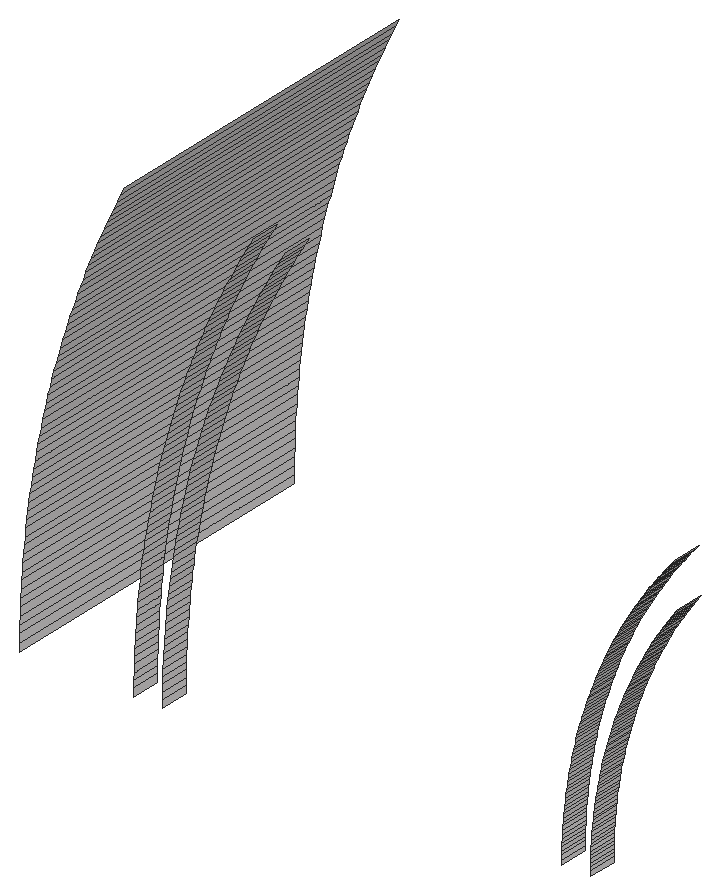
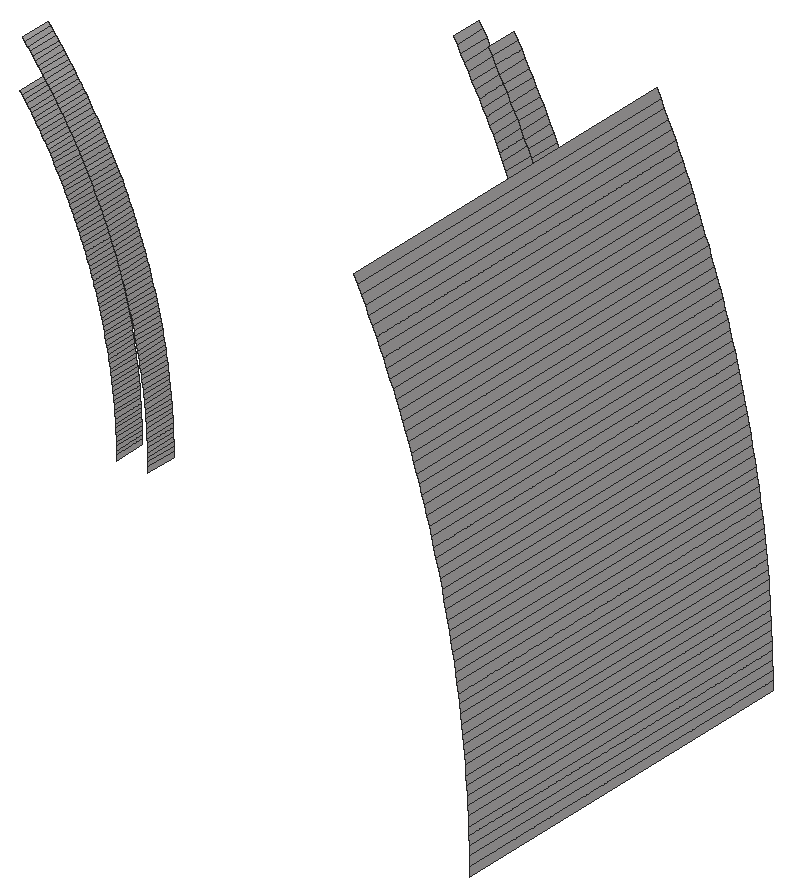
# SketchUp Ruby script. Lengths in inches.
U = 1.inch
M = Sketchup.active_model
def pt(a) = Geom::Point3d.new(a.map { |v| v * U })
def face(e, loops, mat)
  f = e.add_face(loops[0].map { |a| pt(a) })
  loops[1..].each { |l| e.add_face(l.map { |a| pt(a) }).erase! }
  f.material = f.back_material = mat if mat
  f
end
# faces: each face lists its corners as indices into pts; further lists are holes
def faces(e, pts, list, mat = nil) = list.each { |f| face(e, (f[0].is_a?(Array) ? f : [f]).map { |l| l.map { |i| pts[i] } }, mat) }
# xy, xz, yz: faces in a plane at the given z, y or x. An outline is a flat list of corners, or four numbers for a rectangle; further outlines are holes
def ring(l) = l.size == 4 ? [[l[0], l[1]], [l[2], l[1]], [l[2], l[3]], [l[0], l[3]]] : l.each_slice(2).to_a
def flat(e, list, mat, &to3) = list.each { |f| face(e, (f[0].is_a?(Array) ? f : [f]).map { |l| ring(l).map { |u, v| to3.(u, v) } }, mat) }
def xy(e, z, list, mat = nil) = flat(e, list, mat) { |x, y| [x, y, z] }
def xz(e, y, list, mat = nil) = flat(e, list, mat) { |x, z| [x, y, z] }
def yz(e, x, list, mat = nil) = flat(e, list, mat) { |y, z| [x, y, z] }
def lines(e, pts, list) = list.each { |a, b| e.add_line(pt(pts[a]), pt(pts[b])) }
# prism: a flat outline (further loops are holes) pulled along v
def prism(e, loops, v, mat = nil)
  f = face(e, loops, mat); d = Geom::Vector3d.new(v.map { |x| x * U })
  f.pushpull(f.normal.samedirection?(d) ? d.length : -d.length)
end
def box(e, o, s, mat = nil) = prism(e, [[o, [o[0] + s[0], o[1], o[2]], [o[0] + s[0], o[1] + s[1], o[2]], [o[0], o[1] + s[1], o[2]]]], [0, 0, s[2]], mat)
def at(x, y, z, deg = 0) = Geom::Transformation.translation(pt([x, y, z])) * Geom::Transformation.rotation(ORIGIN, Z_AXIS, deg.degrees)
def axes(o, x, y, z) = Geom::Transformation.new([*x, 0, *y, 0, *z, 0, *pt(o).to_a, 1])
def part(name) = M.definitions.add(name)
# library, detail: a bought-in or finely detailed component or shape, given as its bounding box
def library(name, o, s) = part(name).tap { |d| box(d.entities, o, s) }
def detail(e, o, s) = box(e.add_group.entities, o, s)
def put(e, d, t, mat = nil) = e.add_instance(d, t).tap { |i| i.material = mat if mat }
def group(e, t, mat = nil) = e.add_group.tap { |g| g.transformation = t; g.material = mat if mat }.entities
root = M.entities
M.materials.add("[Quartz Light Brown]").color = [215, 212, 212]
yz(root,0,[[38,84,50,84.28],[38,84.28,50,84.57]],"[Quartz Light Brown]")
yz(root,4,[[38,83.99,39,84.25],[38,84.25,39,84.5]],"[Quartz Light Brown]")
yz(root,4.02,[[38,85.01,39,85.26]],"[Quartz Light Brown]")
yz(root,5,[[38,83.99,39,84.24],[38,84.24,39,84.49]],"[Quartz Light Brown]")
yz(root,5.02,[[38,84.97,39,85.22]],"[Quartz Light Brown]")
yz(root,19,[[38,83.96,39,84.13],[38,84.13,39,84.27],[38,84.27,39,84.4]],"[Quartz Light Brown]")
yz(root,19.01,[[38,84.53,39,84.67]],"[Quartz Light Brown]")
yz(root,19.03,[[38,84.93,39,85.07]],"[Quartz Light Brown]")
yz(root,20,[[38,83.96,39,84.125],[38,84.125,39,84.25],[38,84.25,39,84.375]],"[Quartz Light Brown]")
yz(root,20.01,[[38,84.5,39,84.63]],"[Quartz Light Brown]")
yz(root,20.02,[[38,84.75,39,84.88]],"[Quartz Light Brown]")
p = [[19,38,84.4],[19,39,84.4],[19.01,39,84.53],[19.01,38,84.53],[20,39,84.375],[20,38,84.375],
  [20.01,38,84.5],[20.01,39,84.5],[4,38,84.5],[4,39,84.5],[4.01,39,84.75],[4.01,38,84.75],
  [5,39,84.49],[5,38,84.49],[5.01,38,84.73],[5.01,39,84.73],[0,38,84.57],[0.01,38,84.85],
  [0.01,50,84.85],[0,50,84.57],[20.01,39,84.63],[20.01,38,84.63],[20.02,38,84.75],[20.02,39,84.75],
  [5.02,38,84.97],[5.02,39,84.97],[19.01,38,84.67],[19.01,39,84.67],[19.02,39,84.8],[19.02,38,84.8],
  [0.02,38,85.13],[0.02,50,85.13],[4.02,39,85.01],[4.02,38,85.01],[19.03,39,84.93],[19.03,38,84.93],
  [20.02,39,84.88],[20.02,38,84.88],[20.03,38,85],[20.03,39,85],[20.04,38,85.13],[20.04,39,85.13],
  [0.03,38,85.41],[0.03,50,85.41],[19.03,38,85.07],[19.03,39,85.07],[19.04,39,85.2],[19.04,38,85.2],
  [20.05,38,85.26],[20.05,39,85.26],[5.02,39,85.22],[5.02,38,85.22],[5.03,38,85.46],[5.03,39,85.46],
  [19.05,39,85.33],[19.05,38,85.33],[4.02,38,85.26],[4.02,39,85.26],[4.04,39,85.51],[4.04,38,85.51],
  [19.0625,39,85.47],[19.0625,38,85.47],[20.06,38,85.38],[20.06,39,85.38],[0.04,38,85.7],[0.04,50,85.7],
  [20.07,38,85.51],[20.07,39,85.51],[4.05,39,85.76],[4.05,38,85.76],[5.05,38,85.7],[5.05,39,85.7],
  [19.08,39,85.6],[19.08,38,85.6],[20.08,38,85.63],[20.08,39,85.63],[19.09,39,85.73],[19.09,38,85.73],
  [20.1,38,85.76],[20.1,39,85.76],[0.05,38,85.98],[0.05,50,85.98],[5.0625,38,85.95],[5.0625,39,85.95],
  [19.1,39,85.87],[19.1,38,85.87],[4.0625,39,86.01],[4.0625,38,86.01],[20.11,38,85.88],[20.11,39,85.88],
  [5.08,38,86.1875],[5.08,39,86.1875],[19.12,39,86],[19.12,38,86],[20.125,38,86.01],[20.125,39,86.01],
  [0.07,38,86.26],[0.07,50,86.26],[4.08,39,86.26],[4.08,38,86.26],[19.13,39,86.13],[19.13,38,86.13],
  [20.14,38,86.13],[20.14,39,86.13],[19.15,39,86.26],[19.15,38,86.26],[20.16,38,86.25],[20.16,39,86.25],
  [5.1,38,86.43],[5.1,39,86.43],[0.09,38,86.54],[0.09,50,86.54],[4.1,39,86.51],[4.1,38,86.51],
  [19.17,39,86.4],[19.17,38,86.4],[20.18,38,86.38],[20.18,39,86.38],[5.12,38,86.67],[5.12,39,86.67],
  [19.1875,39,86.53],[19.1875,38,86.53],[20.2,38,86.5],[20.2,39,86.5],[0.11,38,86.82],[0.11,50,86.82],
  [4.12,39,86.76],[4.12,38,86.76],[19.21,39,86.66],[19.21,38,86.66],[20.22,38,86.625],[20.22,39,86.625],
  [20.24,38,86.75],[20.24,39,86.75],[5.14,38,86.92],[5.14,39,86.92],[19.23,39,86.79],[19.23,38,86.79],
  [0.13,38,87.11],[0.13,50,87.11],[4.14,39,87.01],[4.14,38,87.01],[19.25,39,86.92],[19.25,38,86.92],
  [20.26,38,86.875],[20.26,39,86.875],[5.16,38,87.16],[5.16,39,87.16],[19.28,39,87.05],[19.28,38,87.05],
  [20.28,38,87],[20.28,39,87],[4.17,39,87.26],[4.17,38,87.26],[20.31,38,87.12],[20.31,39,87.12],
  [0.16,38,87.39],[0.16,50,87.39],[19.3,39,87.19],[19.3,38,87.19],[20.33,38,87.24],[20.33,39,87.24],
  [5.1875,38,87.4],[5.1875,39,87.4],[19.33,39,87.32],[19.33,38,87.32],[20.36,38,87.37],[20.36,39,87.37],
  [4.19,39,87.51],[4.19,38,87.51],[19.35,39,87.45],[19.35,38,87.45],[0.1875,38,87.67],[0.1875,50,87.67],
  [5.21,38,87.64],[5.21,39,87.64],[19.38,39,87.58],[19.38,38,87.58],[20.39,38,87.49],[20.39,39,87.49],
  [4.22,39,87.76],[4.22,38,87.76],[20.41,38,87.61],[20.41,39,87.61],[5.24,38,87.89],[5.24,39,87.89],
  [19.41,39,87.71],[19.41,38,87.71],[20.44,38,87.74],[20.44,39,87.74],[0.22,38,87.95],[0.22,50,87.95],
  [19.4375,39,87.84],[19.4375,38,87.84],[20.47,38,87.86],[20.47,39,87.86],[4.25,39,88.01],[4.25,38,88.01],
  [19.47,39,87.97],[19.47,38,87.97],[5.28,38,88.125],[5.28,39,88.125],[20.5,38,87.98],[20.5,39,87.98],
  [0.25,38,88.23],[0.25,50,88.23],[4.28,39,88.26],[4.28,38,88.26],[19.5,39,88.1],[19.5,38,88.1],
  [20.53,38,88.1],[20.53,39,88.1],[5.31,38,88.37],[5.31,39,88.37],[19.53,39,88.23],[19.53,38,88.23],
  [20.57,38,88.22],[20.57,39,88.22],[0.28,38,88.51],[0.28,50,88.51],[19.57,39,88.36],[19.57,38,88.36],
  [20.6,38,88.34],[20.6,39,88.34],[4.32,39,88.51],[4.32,38,88.51],[20.64,38,88.46],[20.64,39,88.46],
  [5.34,38,88.61],[5.34,39,88.61],[19.6,39,88.49],[19.6,38,88.49],[0.32,38,88.79],[0.32,50,88.79],
  [4.36,39,88.76],[4.36,38,88.76],[19.64,39,88.61],[19.64,38,88.61],[20.67,38,88.58],[20.67,39,88.58],
  [5.38,38,88.85],[5.38,39,88.85],[19.68,39,88.74],[19.68,38,88.74],[20.71,38,88.7],[20.71,39,88.7],
  [19.71,39,88.87],[19.71,38,88.87],[20.74,38,88.82],[20.74,39,88.82],[0.36,38,89.07],[0.36,50,89.07],
  [4.39,39,89.01],[4.39,38,89.01],[5.42,38,89.09],[5.42,39,89.09],[20.78,38,88.94],[20.78,39,88.94],
  [19.75,39,89],[19.75,38,89],[20.82,38,89.0625],[20.82,39,89.0625],[4.43,39,89.25],[4.43,38,89.25],
  [19.79,39,89.125],[19.79,38,89.125],[0.4,38,89.35],[0.4,50,89.35],[5.46,38,89.33],[5.46,39,89.33],
  [19.83,39,89.25],[19.83,38,89.25],[20.86,38,89.18],[20.86,39,89.18],[20.9,38,89.3],[20.9,39,89.3],
  [4.48,39,89.5],[4.48,38,89.5],[5.5,38,89.57],[5.5,39,89.57],[19.875,39,89.38],[19.875,38,89.38],
  [20.95,38,89.42],[20.95,39,89.42],[0.44,38,89.63],[0.44,50,89.63],[19.92,39,89.51],[19.92,38,89.51],
  [20.99,38,89.54],[20.99,39,89.54],[4.52,39,89.75],[4.52,38,89.75],[19.96,39,89.63],[19.96,38,89.63],
  [21.03,38,89.66],[21.03,39,89.66],[0.49,38,89.91],[0.49,50,89.91],[5.55,38,89.81],[5.55,39,89.81],
  [20.01,39,89.76],[20.01,38,89.76],[4.57,39,90],[4.57,38,90],[21.08,38,89.77],[21.08,39,89.77],
  [5.6,38,90.05],[5.6,39,90.05],[20.05,39,89.88],[20.05,38,89.88],[21.125,38,89.89],[21.125,39,89.89],
  [0.54,38,90.1875],[0.54,50,90.1875],[20.1,39,90.01],[20.1,38,90.01],[21.17,38,90.01],[21.17,39,90.01],
  [4.61,39,90.24],[4.61,38,90.24],[5.64,38,90.29],[5.64,39,90.29],[20.15,39,90.13],[20.15,38,90.13],
  [21.22,38,90.12],[21.22,39,90.12],[20.19,39,90.26],[20.19,38,90.26],[21.27,38,90.24],[21.27,39,90.24],
  [0.59,38,90.47],[0.59,50,90.47],[4.66,39,90.49],[4.66,38,90.49],[21.32,38,90.35],[21.32,39,90.35],
  [5.69,38,90.52],[5.69,39,90.52],[20.24,39,90.38],[20.24,38,90.38],[20.29,39,90.51],[20.29,38,90.51],
  [21.37,38,90.47],[21.37,39,90.47],[0.64,38,90.75],[0.64,50,90.75],[4.72,39,90.74],[4.72,38,90.74],
  [5.75,38,90.76],[5.75,39,90.76],[20.35,39,90.63],[20.35,38,90.63],[21.42,38,90.58],[21.42,39,90.58],
  [20.4,39,90.75],[20.4,38,90.75],[21.47,38,90.7],[21.47,39,90.7],[0.69,38,91.02],[0.69,50,91.02],
  [4.77,39,90.98],[4.77,38,90.98],[21.52,38,90.8125],[21.52,39,90.8125],[5.8,38,91],[5.8,39,91],
  [20.45,39,90.875],[20.45,38,90.875],[21.58,38,90.93],[21.58,39,90.93],[20.51,39,91],[20.51,38,91],
  [21.63,38,91.04],[21.63,39,91.04],[0.75,38,91.3],[0.75,50,91.3],[4.83,39,91.23],[4.83,38,91.23],
  [5.86,38,91.24],[5.86,39,91.24],[20.5625,39,91.12],[20.5625,38,91.12],[21.6875,38,91.15],[21.6875,39,91.15],
  [20.62,39,91.24],[20.62,38,91.24],[4.88,39,91.47],[4.88,38,91.47],[5.91,38,91.47],[5.91,39,91.47],
  [20.68,39,91.36],[20.68,38,91.36],[21.74,38,91.26],[21.74,39,91.26],[0.81,38,91.58],[0.81,50,91.58],
  [21.8,38,91.375],[21.8,39,91.375],[20.73,39,91.48],[20.73,38,91.48],[21.86,38,91.49],[21.86,39,91.49],
  [4.94,39,91.71],[4.94,38,91.71],[5.97,38,91.71],[5.97,39,91.71],[20.79,39,91.6],[20.79,38,91.6],
  [21.92,38,91.6],[21.92,39,91.6],[0.87,38,91.85],[0.87,50,91.85],[20.85,39,91.72],[20.85,38,91.72],
  [21.98,38,91.71],[21.98,39,91.71],[5.01,39,91.96],[5.01,38,91.96],[6.04,38,91.94],[6.04,39,91.94],
  [20.91,39,91.84],[20.91,38,91.84],[22.04,38,91.82],[22.04,39,91.82],[20.98,39,91.95],[20.98,38,91.95],
  [22.1,38,91.93],[22.1,39,91.93],[0.93,38,92.13],[0.93,50,92.13],[6.1,38,92.18],[6.1,39,92.18],
  [22.16,38,92.04],[22.16,39,92.04],[5.07,39,92.2],[5.07,38,92.2],[21.04,39,92.07],[21.04,38,92.07],
  [22.23,38,92.14],[22.23,39,92.14],[0.99,38,92.4],[0.99,50,92.4],[21.1,39,92.19],[21.1,38,92.19],
  [22.29,38,92.25],[22.29,39,92.25],[5.13,39,92.44],[5.13,38,92.44],[6.16,38,92.41],[6.16,39,92.41],
  [21.17,39,92.31],[21.17,38,92.31],[21.23,39,92.42],[21.23,38,92.42],[22.36,38,92.36],[22.36,39,92.36],
  [1.0625,38,92.68],[1.0625,50,92.68],[5.2,39,92.6875],[5.2,38,92.6875],[6.23,38,92.65],[6.23,39,92.65],
  [21.3,39,92.54],[21.3,38,92.54],[22.42,38,92.47],[22.42,39,92.47],[21.37,39,92.65],[21.37,38,92.65],
  [22.49,38,92.57],[22.49,39,92.57],[6.3,38,92.88],[6.3,39,92.88],[22.56,38,92.68],[22.56,39,92.68],
  [1.13,38,92.95],[1.13,50,92.95],[5.27,39,92.93],[5.27,38,92.93],[21.4375,39,92.77],[21.4375,38,92.77],
  [22.63,38,92.78],[22.63,39,92.78],[21.51,39,92.88],[21.51,38,92.88],[22.7,38,92.89],[22.7,39,92.89],
  [5.34,39,93.17],[5.34,38,93.17],[6.37,38,93.12],[6.37,39,93.12],[21.58,39,93],[21.58,38,93],
  [22.77,38,92.99],[22.77,39,92.99],[1.2,38,93.23],[1.2,50,93.23],[21.65,39,93.11],[21.65,38,93.11],
  [22.84,38,93.1],[22.84,39,93.1],[6.44,38,93.35],[6.44,39,93.35],[21.72,39,93.22],[21.72,38,93.22],
  [22.91,38,93.2],[22.91,39,93.2],[1.28,38,93.5],[1.28,50,93.5],[5.41,39,93.41],[5.41,38,93.41],
  [21.79,39,93.33],[21.79,38,93.33],[22.98,38,93.3],[22.98,39,93.3],[6.52,38,93.58],[6.52,39,93.58],
  [21.87,39,93.44],[21.87,38,93.44],[23.06,38,93.4],[23.06,39,93.4],[5.49,39,93.65],[5.49,38,93.65],
  [21.94,39,93.56],[21.94,38,93.56],[1.35,38,93.77],[1.35,50,93.77],[5.57,39,93.89],[5.57,38,93.89],
  [6.59,38,93.8125],[6.59,39,93.8125],[22.02,39,93.67],[22.02,38,93.67],[22.09,39,93.78],[22.09,38,93.78],
  [1.43,38,94.04],[1.43,50,94.04],[6.67,38,94.04],[6.67,39,94.04],[22.17,39,93.88],[22.17,38,93.88],
  [5.64,39,94.13],[5.64,38,94.13],[22.25,39,93.99],[22.25,38,93.99],[1.51,38,94.31],[1.51,50,94.31],
  [6.75,38,94.27],[6.75,39,94.27],[22.33,39,94.1],[22.33,38,94.1],[5.73,39,94.37],[5.73,38,94.37],
  [22.41,39,94.21],[22.41,38,94.21],[22.49,39,94.3125],[22.49,38,94.3125],[1.59,38,94.59],[1.59,50,94.59],
  [6.83,38,94.5],[6.83,39,94.5],[22.57,39,94.42],[22.57,38,94.42],[5.81,39,94.6],[5.81,38,94.6],
  [22.65,39,94.52],[22.65,38,94.52],[6.92,38,94.73],[6.92,39,94.73],[22.73,39,94.63],[22.73,38,94.63],
  [1.68,38,94.86],[1.68,50,94.86],[5.89,39,94.84],[5.89,38,94.84],[22.82,39,94.73],[22.82,38,94.73],
  [7,38,94.96],[7,39,94.96],[22.9,39,94.84],[22.9,38,94.84],[5.98,39,95.08],[5.98,38,95.08],
  [22.99,39,94.9375],[22.99,38,94.9375],[1.76,38,95.125],[1.76,50,95.125],[7.09,38,95.19],[7.09,39,95.19],
  [1.85,38,95.39],[1.85,50,95.39],[6.07,39,95.3125],[6.07,38,95.3125],[7.18,38,95.41],[7.18,39,95.41],
  [6.16,39,95.55],[6.16,38,95.55],[1.94,38,95.66],[1.94,50,95.66],[7.27,38,95.64],[7.27,39,95.64],
  [6.25,39,95.78],[6.25,38,95.78],[7.36,38,95.86],[7.36,39,95.86],[2.03,38,95.93],[2.03,50,95.93],
  [6.34,39,96.01],[6.34,38,96.01],[2.13,38,96.19],[2.13,50,96.19],[7.45,38,96.09],[7.45,39,96.09],
  [6.4375,39,96.25],[6.4375,38,96.25],[7.55,38,96.3125],[7.55,39,96.3125],[2.23,38,96.46],[2.23,50,96.46],
  [6.53,39,96.48],[6.53,38,96.48],[7.65,38,96.53],[7.65,39,96.53],[2.32,38,96.73],[2.32,50,96.73],
  [6.63,39,96.71],[6.63,38,96.71],[7.75,38,96.76],[7.75,39,96.76],[2.42,38,96.99],[2.42,50,96.99],
  [6.73,39,96.9375],[6.73,38,96.9375],[7.85,38,96.98],[7.85,39,96.98],[6.84,39,97.17],[6.84,38,97.17],
  [2.53,38,97.25],[2.53,50,97.25],[7.95,38,97.2],[7.95,39,97.2],[6.9375,39,97.4],[6.9375,38,97.4],
  [8.05,38,97.42],[8.05,39,97.42],[2.63,38,97.51],[2.63,50,97.51],[7.05,39,97.625],[7.05,38,97.625],
  [8.16,38,97.64],[8.16,39,97.64],[2.74,38,97.78],[2.74,50,97.78],[7.15,39,97.85],[7.15,38,97.85],
  [8.27,38,97.86],[8.27,39,97.86],[2.85,38,98.04],[2.85,50,98.04],[7.26,39,98.08],[7.26,38,98.08],
  [8.38,38,98.07],[8.38,39,98.07],[2.96,38,98.3],[2.96,50,98.3],[7.375,39,98.3],[7.375,38,98.3],
  [8.49,38,98.29],[8.49,39,98.29],[3.07,38,98.56],[3.07,50,98.56],[7.49,39,98.53],[7.49,38,98.53],
  [8.6,38,98.51],[8.6,39,98.51],[7.6,39,98.75],[7.6,38,98.75],[8.72,38,98.72],[8.72,39,98.72],
  [3.1875,38,98.81],[3.1875,50,98.81],[8.83,38,98.93],[8.83,39,98.93],[3.31,38,99.07],[3.31,50,99.07],
  [7.72,39,98.97],[7.72,38,98.97],[8.95,38,99.15],[8.95,39,99.15],[7.84,39,99.2],[7.84,38,99.2],
  [3.43,38,99.33],[3.43,50,99.33],[9.07,38,99.36],[9.07,39,99.36],[7.96,39,99.42],[7.96,38,99.42],
  [3.55,38,99.58],[3.55,50,99.58],[8.08,39,99.64],[8.08,38,99.64],[9.19,38,99.57],[9.19,39,99.57],
  [3.67,38,99.84],[3.67,50,99.84],[8.2,39,99.85],[8.2,38,99.85],[9.32,38,99.78],[9.32,39,99.78]]
faces(root,p,[[0,1,2,3],[4,5,6,7],[8,9,10,11],[12,13,14,15],[16,17,18,19],[20,21,22,23],[15,14,24,25],[26,27,28,29],
  [17,30,31,18],[11,10,32,33],[29,28,34,35],[36,37,38,39],[39,38,40,41],[30,42,43,31],[44,45,46,47],[41,40,48,49],
  [50,51,52,53],[47,46,54,55],[56,57,58,59],[55,54,60,61],[49,48,62,63],[42,64,65,43],[63,62,66,67],[59,58,68,69],
  [53,52,70,71],[61,60,72,73],[67,66,74,75],[73,72,76,77],[75,74,78,79],[64,80,81,65],[71,70,82,83],[77,76,84,85],
  [69,68,86,87],[79,78,88,89],[83,82,90,91],[85,84,92,93],[89,88,94,95],[80,96,97,81],[87,86,98,99],[93,92,100,101],
  [95,94,102,103],[101,100,104,105],[103,102,106,107],[91,90,108,109],[96,110,111,97],[99,98,112,113],[105,104,114,115],[107,106,116,117],
  [109,108,118,119],[115,114,120,121],[117,116,122,123],[110,124,125,111],[113,112,126,127],[121,120,128,129],[123,122,130,131],[131,130,132,133],
  [119,118,134,135],[129,128,136,137],[124,138,139,125],[127,126,140,141],[137,136,142,143],[133,132,144,145],[135,134,146,147],[143,142,148,149],
  [145,144,150,151],[141,140,152,153],[151,150,154,155],[138,156,157,139],[149,148,158,159],[155,154,160,161],[147,146,162,163],[159,158,164,165],
  [161,160,166,167],[153,152,168,169],[165,164,170,171],[156,172,173,157],[163,162,174,175],[171,170,176,177],[167,166,178,179],[169,168,180,181],
  [179,178,182,183],[175,174,184,185],[177,176,186,187],[183,182,188,189],[172,190,191,173],[187,186,192,193],[189,188,194,195],[181,180,196,197],
  [193,192,198,199],[185,184,200,201],[195,194,202,203],[190,204,205,191],[197,196,206,207],[199,198,208,209],[203,202,210,211],[201,200,212,213],
  [209,208,214,215],[211,210,216,217],[204,218,219,205],[215,214,220,221],[217,216,222,223],[207,206,224,225],[223,222,226,227],[213,212,228,229],
  [221,220,230,231],[218,232,233,219],[225,224,234,235],[231,230,236,237],[227,226,238,239],[229,228,240,241],[237,236,242,243],[239,238,244,245],
  [243,242,246,247],[245,244,248,249],[232,250,251,233],[235,234,252,253],[241,240,254,255],[249,248,256,257],[247,246,258,259],[257,256,260,261],
  [253,252,262,263],[259,258,264,265],[250,266,267,251],[255,254,268,269],[265,264,270,271],[261,260,272,273],[273,272,274,275],[263,262,276,277],
  [269,268,278,279],[271,270,280,281],[275,274,282,283],[266,284,285,267],[281,280,286,287],[283,282,288,289],[277,276,290,291],[287,286,292,293],
  [289,288,294,295],[284,296,297,285],[279,278,298,299],[293,292,300,301],[291,290,302,303],[295,294,304,305],[299,298,306,307],[301,300,308,309],
  [305,304,310,311],[296,312,313,297],[309,308,314,315],[311,310,316,317],[303,302,318,319],[307,306,320,321],[315,314,322,323],[317,316,324,325],
  [323,322,326,327],[325,324,328,329],[312,330,331,313],[319,318,332,333],[329,328,334,335],[321,320,336,337],[327,326,338,339],[339,338,340,341],
  [335,334,342,343],[330,344,345,331],[333,332,346,347],[337,336,348,349],[341,340,350,351],[343,342,352,353],[351,350,354,355],[353,352,356,357],
  [344,358,359,345],[347,346,360,361],[357,356,362,363],[349,348,364,365],[355,354,366,367],[363,362,368,369],[367,366,370,371],[369,368,372,373],
  [358,374,375,359],[361,360,376,377],[365,364,378,379],[371,370,380,381],[373,372,382,383],[381,380,384,385],[377,376,386,387],[379,378,388,389],
  [385,384,390,391],[383,382,392,393],[374,394,395,375],[393,392,396,397],[391,390,398,399],[397,396,400,401],[387,386,402,403],[389,388,404,405],
  [399,398,406,407],[401,400,408,409],[394,410,411,395],[407,406,412,413],[409,408,414,415],[403,402,416,417],[405,404,418,419],[413,412,420,421],
  [415,414,422,423],[421,420,424,425],[423,422,426,427],[410,428,429,411],[419,418,430,431],[427,426,432,433],[417,416,434,435],[425,424,436,437],
  [433,432,438,439],[428,440,441,429],[437,436,442,443],[439,438,444,445],[435,434,446,447],[431,430,448,449],[443,442,450,451],[451,450,452,453],
  [445,444,454,455],[440,456,457,441],[447,446,458,459],[449,448,460,461],[453,452,462,463],[455,454,464,465],[463,462,466,467],[465,464,468,469],
  [461,460,470,471],[469,468,472,473],[456,474,475,457],[459,458,476,477],[467,466,478,479],[473,472,480,481],[479,478,482,483],[481,480,484,485],
  [477,476,486,487],[471,470,488,489],[483,482,490,491],[485,484,492,493],[474,494,495,475],[491,490,496,497],[493,492,498,499],[489,488,500,501],
  [497,496,502,503],[499,498,504,505],[494,506,507,495],[487,486,508,509],[503,502,510,511],[505,504,512,513],[501,500,514,515],[511,510,516,517],
  [513,512,518,519],[509,508,520,521],[517,516,522,523],[506,524,525,507],[521,520,526,527],[515,514,528,529],[523,522,530,531],[531,530,532,533],
  [524,534,535,525],[529,528,536,537],[533,532,538,539],[527,526,540,541],[539,538,542,543],[534,544,545,535],[537,536,546,547],[543,542,548,549],
  [541,540,550,551],[549,548,552,553],[553,552,554,555],[544,556,557,545],[547,546,558,559],[555,554,560,561],[551,550,562,563],[561,560,564,565],
  [559,558,566,567],[565,564,568,569],[556,570,571,557],[563,562,572,573],[569,568,574,575],[567,566,576,577],[575,574,578,579],[573,572,580,581],
  [579,578,582,583],[570,584,585,571],[577,576,586,587],[584,588,589,585],[581,580,590,591],[587,586,592,593],[591,590,594,595],[588,596,597,589],
  [593,592,598,599],[595,594,600,601],[599,598,602,603],[596,604,605,597],[601,600,606,607],[604,608,609,605],[603,602,610,611],[607,606,612,613],
  [611,610,614,615],[608,616,617,609],[613,612,618,619],[615,614,620,621],[616,622,623,617],[619,618,624,625],[621,620,626,627],[622,628,629,623],
  [625,624,630,631],[627,626,632,633],[631,630,634,635],[628,636,637,629],[633,632,638,639],[635,634,640,641],[639,638,642,643],[636,644,645,637],
  [641,640,646,647],[643,642,648,649],[644,650,651,645],[647,646,652,653],[649,648,654,655],[650,656,657,651],[653,652,658,659],[655,654,660,661],
  [656,662,663,657],[659,658,664,665],[661,660,666,667],[662,668,669,663],[665,664,670,671],[667,666,672,673],[671,670,674,675],[673,672,676,677],
  [668,678,679,669],[677,676,680,681],[678,682,683,679],[675,674,684,685],[681,680,686,687],[685,684,688,689],[682,690,691,683],[687,686,692,693],
  [689,688,694,695],[690,696,697,691],[695,694,698,699],[693,692,700,701],[696,702,703,697],[699,698,704,705],[701,700,706,707]],"[Quartz Light Brown]")
